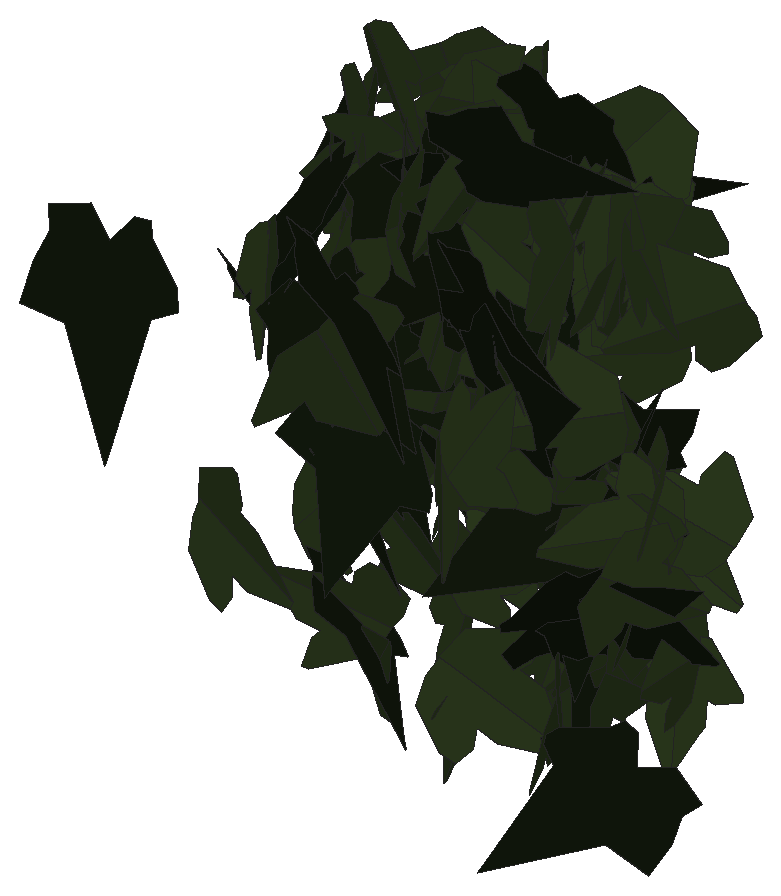
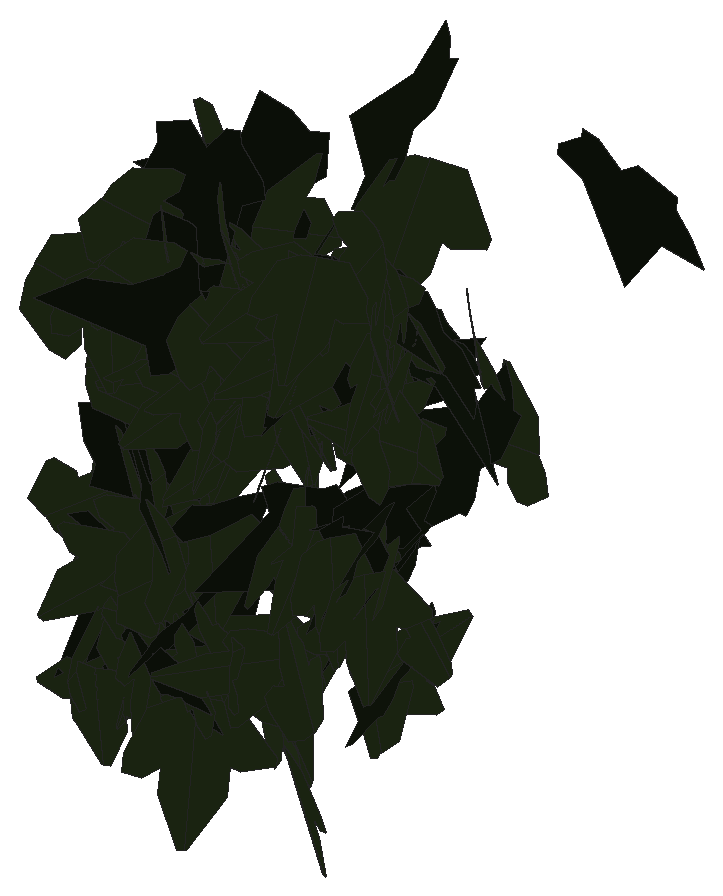
# SketchUp Ruby script. Lengths in inches.
U = 1.inch
M = Sketchup.active_model
def pt(a) = Geom::Point3d.new(a.map { |v| v * U })
def face(e, loops, mat)
  f = e.add_face(loops[0].map { |a| pt(a) })
  loops[1..].each { |l| e.add_face(l.map { |a| pt(a) }).erase! }
  f.material = f.back_material = mat if mat
  f
end
# faces: each face lists its corners as indices into pts; further lists are holes
def faces(e, pts, list, mat = nil) = list.each { |f| face(e, (f[0].is_a?(Array) ? f : [f]).map { |l| l.map { |i| pts[i] } }, mat) }
# xy, xz, yz: faces in a plane at the given z, y or x. An outline is a flat list of corners, or four numbers for a rectangle; further outlines are holes
def ring(l) = l.size == 4 ? [[l[0], l[1]], [l[2], l[1]], [l[2], l[3]], [l[0], l[3]]] : l.each_slice(2).to_a
def flat(e, list, mat, &to3) = list.each { |f| face(e, (f[0].is_a?(Array) ? f : [f]).map { |l| ring(l).map { |u, v| to3.(u, v) } }, mat) }
def xy(e, z, list, mat = nil) = flat(e, list, mat) { |x, y| [x, y, z] }
def xz(e, y, list, mat = nil) = flat(e, list, mat) { |x, z| [x, y, z] }
def yz(e, x, list, mat = nil) = flat(e, list, mat) { |y, z| [x, y, z] }
def lines(e, pts, list) = list.each { |a, b| e.add_line(pt(pts[a]), pt(pts[b])) }
# prism: a flat outline (further loops are holes) pulled along v
def prism(e, loops, v, mat = nil)
  f = face(e, loops, mat); d = Geom::Vector3d.new(v.map { |x| x * U })
  f.pushpull(f.normal.samedirection?(d) ? d.length : -d.length)
end
def box(e, o, s, mat = nil) = prism(e, [[o, [o[0] + s[0], o[1], o[2]], [o[0] + s[0], o[1] + s[1], o[2]], [o[0], o[1] + s[1], o[2]]]], [0, 0, s[2]], mat)
def at(x, y, z, deg = 0) = Geom::Transformation.translation(pt([x, y, z])) * Geom::Transformation.rotation(ORIGIN, Z_AXIS, deg.degrees)
def axes(o, x, y, z) = Geom::Transformation.new([*x, 0, *y, 0, *z, 0, *pt(o).to_a, 1])
def part(name) = M.definitions.add(name)
# library, detail: a bought-in or finely detailed component or shape, given as its bounding box
def library(name, o, s) = part(name).tap { |d| box(d.entities, o, s) }
def detail(e, o, s) = box(e.add_group.entities, o, s)
def put(e, d, t, mat = nil) = e.add_instance(d, t).tap { |i| i.material = mat if mat }
def group(e, t, mat = nil) = e.add_group.tap { |g| g.transformation = t; g.material = mat if mat }.entities
root = M.entities
M.materials.add("efeu1").color = [18, 25, 13]
M.materials.add("efeu2").color = [43, 57, 29]
c1 = part("ivyleaf_10")
p = [[0,0.5,-0.03],[-0.0625,2.02,-0.43],[-0.19,2.01,-0.46],[-0.54,1.05,-0.29],[-0.52,0.625,-0.18],[-0.83,0.76,-0.28],
  [-1.16,0.64,-0.33],[-1.15,0.33,-0.24],[-0.77,-0.39,0.02],[-0.3,-0.51,0.16],[0.04,-0.48,0.23],[-0.02,2.01,-0.4375],
  [-0.06,2.01,-0.43],[0.04,-0.49,0.23],[0.67,-0.49,0.14],[1.38,0.36,-0.2],[1.375,0.51,-0.24],[0.81,0.65,-0.19],
  [0.62,0.59,-0.15],[0.6,1.09,-0.28],[0.5,1.23,-0.31]]
faces(c1.entities,p,[[0,1,2,3,4,5,6,7,8,9,10],[11,12,0,13,14,15,16,17,18,19,20]],"efeu2")
c2 = part("ivyleaf_9")
p = [[1.54,2.16,1.25],[1.36,2.04,1.19],[-0.21,0.99,0.68],[-0.71,1.11,0.82],[-0.85,0.86,0.67],[-0.8,0.17,0.21],
  [-0.9,-0.01,0.1],[-0.67,-0.16,-0.02],[-0.08,-0.08,-0.05],[-0.03,-0.6,-0.4],[0.65,-0.88,-0.66],[0.83,-0.6,-0.49],
  [1.29,-0.42,-0.43],[1.8125,-0.07,-0.26],[1.21,0.44,0.15]]
faces(c2.entities,p,[[0,1,2,3,4,5,6,7,8,9,10,11,12,13,14]],"efeu1")
put(root,c1,axes([519.33,135.79,170.69],[-0.23266,0.62806,-0.07451],[0.02428,-0.07046,-0.66976],[-0.63199,-0.23391,0.0017]))
put(root,c1,axes([519.5,136.4375,167.12],[-0.25165,-0.66074,-0.04821],[0.01912,0.04431,-0.70703],[0.66222,-0.25237,0.00209]))
put(root,c1,axes([519.49,136.15,169.66],[-0.01709,-0.51856,0.5127],[0.02176,-0.51297,-0.51812],[0.7289,0.00315,0.02749]))
put(root,c1,axes([519.18,136.53,171.21],[0.40833,-0.42792,0.4417],[0.33385,-0.29103,-0.59058],[0.51648,0.52643,0.03254]))
put(root,c2,axes([519.73,134.51,170.41],[-0.53157,0.4474,-0.34863],[-0.26413,0.22758,0.69478],[0.50194,0.59357,-0.00361]))
put(root,c2,axes([518.93,134.71,168.71],[0.30061,-0.52854,0.55192],[0.33869,-0.43951,-0.60536],[0.68502,0.44924,0.05711]))
put(root,c2,axes([519.96,134.43,170.3],[-0.45095,0.63568,0.03637],[-0.02109,0.02963,-0.77938],[-0.63637,-0.45144,0.00006]))
put(root,c2,axes([519.4,130.97,171.44],[-0.62902,-0.2297,-0.64286],[0.60631,0.21376,-0.66963],[0.31374,-0.87364,0.00518]))
put(root,c1,axes([519.39,135.875,171.5],[-0.28758,0.30723,-0.51733],[0.2824,-0.43739,-0.41674],[-0.5313,-0.39878,0.05851]))
put(root,c1,axes([519.67,135.97,170.63],[-0.01143,-0.49947,-0.4386],[0.05584,0.4364,-0.49841],[0.66236,-0.04541,0.03445]))
put(root,c1,axes([519.42,134.04,170.125],[0.46577,-0.26689,0.42385],[0.35567,-0.2313,-0.53649],[0.35268,0.58574,-0.01872]))
put(root,c1,axes([519.34,135.15,165.76],[0.42672,-0.23414,-0.46095],[0.40158,-0.22632,0.48672],[-0.32562,-0.58596,-0.0038]))
put(root,c1,axes([519.28,136.04,169.49],[-0.02495,-0.08833,0.66389],[0.61696,0.25549,0.05717],[-0.26062,0.61327,0.0718]))
put(root,c1,axes([520.23,135.5,171.12],[0.3467,0.09818,-0.56949],[-0.57753,0.08246,-0.33738],[0.02053,0.66161,0.12656]))
put(root,c1,axes([519.9375,136.61,167.62],[-0.19817,-0.6743,-0.05006],[0.00873,0.04961,-0.70279],[0.6761,-0.19829,-0.0056]))
put(root,c1,axes([519.99,135.5625,169.02],[-0.38877,-0.52025,-0.20837],[-0.12833,-0.16422,0.64945],[-0.54554,0.40938,-0.00429]))
put(root,c1,axes([519.68,136,166.91],[-0.37064,0.21017,0.64179],[0.50889,-0.39435,0.42303],[0.44396,0.6275,0.05089]))
put(root,c1,axes([519.8125,136,172.27],[-0.4826,0.31295,-0.40914],[0.31544,-0.26367,-0.57377],[-0.40722,-0.57513,0.04042]))
put(root,c2,axes([519.75,135.83,166.98],[0.37466,-0.64244,-0.187],[-0.09447,0.16138,-0.7437],[0.6624,0.38638,-0.0003]))
put(root,c2,axes([520.1875,136.2,168.02],[-0.41218,-0.63662,0.24656],[-0.11009,-0.22226,-0.75792],[0.67377,-0.42577,0.02699]))
put(root,c1,axes([520.59,134.72,164.89],[-0.32035,-0.19606,-0.6035],[-0.51146,-0.32036,0.37557],[-0.37558,0.60349,0.0033]))
put(root,c2,axes([519.79,136.33,167.6],[0.42774,-0.61794,0.13653],[0.08201,-0.10927,-0.75153],[0.62751,0.4355,0.00516]))
put(root,c1,axes([520.25,136.72,171.97],[-0.43152,-0.5374,-0.18953],[0.13459,0.1349,-0.68893],[0.55373,-0.45159,0.01975]))
put(root,c1,axes([520.15,137,165.48],[0.19906,-0.67643,-0.07018],[0.03815,-0.0619,0.70486],[-0.67899,-0.20179,0.01903]))
put(root,c1,axes([519.83,136.18,166.74],[-0.24481,-0.21364,0.74665],[0.58059,0.4696,0.32472],[-0.51579,0.62999,0.01115]))
put(root,c1,axes([520.31,136.56,167.92],[-0.20784,-0.53843,-0.40911],[0.14041,0.38431,-0.57712],[0.66148,-0.25075,-0.00604]))
put(root,c1,axes([520.23,136.3,171.27],[-0.52379,-0.43811,-0.3686],[0.27047,0.25099,-0.68266],[0.50464,-0.58926,-0.01671]))
put(root,c1,axes([520.57,136.03,167.3],[-0.40169,-0.57434,0.1525],[-0.08114,-0.12933,-0.70083],[0.58868,-0.40973,0.00746]))
put(root,c1,axes([520.41,137.14,168.17],[-0.00629,0.59882,-0.47127],[-0.05118,-0.47056,-0.59723],[-0.76031,0.02672,0.0441]))
put(root,c2,axes([520.26,134.26,169.59],[0.17214,-0.5842,-0.53926],[-0.08366,0.53539,-0.60671],[0.79063,0.18384,0.05321]))
put(root,c2,axes([520.03,134.69,167.17],[0.42398,-0.59008,0.34279],[0.18551,-0.28871,-0.72643],[0.65673,0.46251,-0.01611]))
put(root,c1,axes([520.55,136.64,164.2],[0.5799,-0.53773,-0.01596],[-0.01344,0.00898,-0.79084],[0.5378,0.58005,-0.00255]))
put(root,c2,axes([520.14,136.29,167.96],[0.04751,-0.01877,-0.7655],[0.33342,0.69096,0.00375],[0.68933,-0.33292,0.05094]))
put(root,c2,axes([520.17,134.91,165.01],[0.34293,-0.66391,0.2397],[0.12675,-0.20423,-0.74702],[0.69438,0.36516,0.01799]))
put(root,c1,axes([520.53,134.8125,164.08],[-0.48234,0.13534,0.4645],[0.4358,-0.16334,0.50012],[0.21013,0.64941,0.02899]))
put(root,c1,axes([521.02,136.16,170],[0.58753,-0.19388,-0.2971],[-0.27123,0.125,-0.61795],[0.22867,0.6464,0.03039]))
put(root,c2,axes([520.65,135.58,171],[0.0571,-0.5406,-0.59781],[-0.08751,0.59161,-0.54334],[0.80123,0.10314,-0.01674]))
put(root,c1,axes([520.24,132.02,167.34],[0.15126,-0.04534,0.82537],[0.82533,-0.03832,-0.15336],[0.04591,0.83824,0.03764]))
put(root,c1,axes([520.62,136.52,171.72],[-0.52511,-0.03265,-0.43392],[0.43514,-0.04425,-0.52325],[-0.00311,-0.67976,0.0549]))
put(root,c1,axes([520.78,136.22,170.46],[0.00261,0.04743,0.71943],[0.04134,0.71825,-0.0475],[-0.71981,0.04142,-0.00012]))
put(root,c1,axes([520.72,135.35,171.3125],[-0.10421,0.29403,-0.60238],[0.20064,-0.56798,-0.31195],[-0.63957,-0.22609,0.00029]))
put(root,c1,axes([521.1,134.81,170.04],[-0.04828,-0.35832,0.57818],[-0.09626,-0.5702,-0.36142],[0.67336,-0.1072,-0.01021]))
put(root,c2,axes([520.83,134.53,167.74],[-0.18099,-0.75598,0.18495],[-0.02625,-0.18385,-0.77716],[0.77783,-0.18211,0.01681]))
put(root,c1,axes([521.15,134.71,170.73],[-0.08628,0.16478,0.66581],[-0.32591,0.58061,-0.18592],[-0.60352,-0.3371,0.00522]))
put(root,c1,axes([520.73,136.46,171.71],[-0.24232,-0.2459,-0.64819],[0.44152,0.47465,-0.34512],[0.53449,-0.50357,-0.00878]))
put(root,c2,axes([520.39,135.45,170.53],[0.26919,0.35615,-0.71425],[0.43465,0.56678,0.44643],[0.66939,-0.51125,-0.00265]))
put(root,c1,axes([521.29,135.26,169.54],[0.14655,-0.22206,-0.63963],[-0.29604,0.56755,-0.26487],[0.60892,0.32937,0.02517]))
put(root,c1,axes([521.49,134.66,166.05],[-0.40606,0.21039,-0.52397],[-0.49986,0.1662,0.45411],[0.26259,0.64173,0.05418]))
put(root,c2,axes([520.93,136.74,169.06],[-0.00659,-0.28089,0.71899],[-0.01168,-0.7189,-0.28096],[0.77182,-0.01327,0.00189]))
put(root,c1,axes([520.82,136.2,167.51],[0.02241,-0.05749,0.67477],[0.55204,-0.38952,-0.05152],[0.39227,0.55145,0.03395]))
put(root,c1,axes([521.31,136.14,167.93],[0.35311,-0.57726,-0.18258],[-0.09782,0.15419,-0.67669],[0.59749,0.3664,-0.00288]))
put(root,c2,axes([520.93,136.83,170.57],[0.14438,-0.73635,0.28054],[0.04963,-0.27615,-0.75037],[0.78642,0.15262,-0.00415]))
put(root,c1,axes([521.51,135.6,169.69],[-0.27167,-0.78398,0.10246],[-0.02615,-0.09937,-0.82968],[0.79021,-0.27282,0.00777]))
put(root,c1,axes([520.98,136.15,165.02],[-0.2513,-0.10464,0.59052],[0.5522,0.20942,0.2721],[-0.23397,0.60664,0.00793]))
put(root,c1,axes([521.88,136.28,168.89],[0.09787,0.35208,0.67435],[-0.27451,-0.61775,0.36237],[0.70947,-0.28759,0.04719]))
put(root,c1,axes([521.95,136.65,165.45],[0.41481,-0.11474,0.54991],[-0.5213,0.17609,0.42996],[-0.20932,-0.66593,0.01895]))
put(root,c1,axes([521.24,136.52,165.57],[0.16282,-0.1407,-0.73673],[0.58167,0.49964,0.03313],[0.47353,-0.56537,0.21262]))
put(root,c2,axes([521.48,135.14,169.55],[-0.17973,-0.10602,0.805],[0.68086,0.42953,0.20858],[-0.44238,0.70415,-0.00604]))
put(root,c1,axes([522.02,136.78,170.73],[-0.26971,-0.44167,0.43769],[-0.226,-0.37484,-0.5175],[0.57928,-0.35188,0.00189]))
put(root,c1,axes([521.62,136.79,172.21],[0.47707,-0.32733,0.41814],[0.33292,-0.25354,-0.57833],[0.4137,0.58151,-0.01678]))
put(root,c1,axes([521.74,134.85,167.43],[-0.1686,0.55926,-0.41859],[0.11803,-0.40161,-0.58412],[-0.68852,-0.2058,0.00237]))
put(root,c1,axes([521.92,135.29,164.2],[0.14994,-0.65208,0.19783],[0.04164,-0.19342,-0.66909],[0.68015,0.15559,-0.00265]))
put(root,c1,axes([521.83,135.52,171.71],[0.00181,-0.366,0.7582],[0.21242,-0.73347,-0.35457],[0.81468,0.19206,0.09077]))
put(root,c1,axes([522.16,135.9375,170.8125],[0.08029,0.14766,-0.67656],[-0.43865,-0.51618,-0.16471],[-0.53584,0.44468,0.03346]))
put(root,c1,axes([521.51,136.07,171.17],[-0.07759,-0.05338,-0.76196],[0.67215,-0.36856,-0.04262],[-0.36282,-0.67138,0.08398]))
put(root,c1,axes([522.23,135.92,169.26],[-0.15605,0.4272,0.60679],[-0.28096,0.53989,-0.45236],[-0.68685,-0.31791,0.04718]))
put(root,c2,axes([521.75,135.12,170.82],[0.45549,-0.63563,-0.11104],[-0.06315,0.09135,-0.78198],[0.64216,0.45984,0.00186]))
put(root,c1,axes([522.29,136.73,164.26],[-0.62581,-0.54341,-0.04469],[0.03437,0.02858,-0.82881],[0.54416,-0.62676,0.00095]))
put(root,c1,axes([522.17,131.91,170.6],[-0.3289,-0.76075,-0.42534],[0.20515,0.37428,-0.82805],[0.8471,-0.38601,0.03539]))
put(root,c1,axes([522.42,136.16,171.07],[0.75128,-0.00861,-0.03698],[-0.03689,0.00752,-0.75129],[0.00897,0.75215,0.00708]))
put(root,c1,axes([522.1875,134.67,164.59],[0.29857,0.42412,0.62452],[0.30949,0.54379,-0.51725],[-0.68856,0.42832,0.03831]))
put(root,c1,axes([522.69,135.91,166.86],[-0.54968,-0.45949,0.07673],[-0.06041,-0.04738,-0.71643],[0.46192,-0.55298,-0.00238]))
put(root,c1,axes([522.14,136.88,165.18],[0.3626,-0.17479,0.55642],[0.5525,-0.10693,-0.39363],[0.18682,0.65548,0.08416]))
put(root,c2,axes([522.89,136.05,166.71],[-0.47757,-0.42822,0.46382],[-0.35102,-0.30324,-0.6414],[0.52467,-0.59266,-0.00694]))
put(root,c1,axes([522.33,136.54,169.45],[-0.44851,-0.13524,-0.49031],[0.46838,0.14502,-0.46845],[0.19828,-0.64848,-0.00251]))
put(root,c1,axes([522.14,135.07,170.6875],[0.30306,0.07748,0.6264],[0.58938,0.21391,-0.31161],[-0.22585,0.66217,0.02737]))
put(root,c2,axes([522.84,135.77,172.67],[0.49521,0.23706,-0.52645],[-0.47962,-0.21721,-0.54897],[-0.32142,0.68935,0.00807]))
put(root,c2,axes([522.42,136.72,166.03],[0.0477,-0.81547,0.17255],[0.0191,-0.17172,-0.81681],[0.8333,0.05062,0.00884]))
put(root,c2,axes([522.71,135.41,170.07],[-0.67627,-0.11085,-0.41353],[0.40664,0.07549,-0.68525],[0.13391,-0.78908,-0.00747]))
put(root,c1,axes([522.25,136.54,169.72],[-0.18472,-0.05142,-0.72029],[0.70102,0.16566,-0.19161],[0.17331,-0.72491,0.0073]))
put(root,c2,axes([522.11,134.86,171.97],[0.44229,-0.04822,0.63431],[0.62875,-0.08427,-0.44482],[0.09668,0.76867,-0.00898]))
put(root,c1,axes([522.73,135.09,167.86],[0.03226,0.0851,0.77042],[-0.09607,0.76558,-0.08055],[-0.76913,-0.09206,0.04237]))
put(root,c1,axes([522.45,135.5,169.17],[-0.32877,-0.02586,-0.57333],[0.55372,-0.18805,-0.30904],[-0.15092,-0.63359,0.11512]))
put(root,c2,axes([522.83,136.86,165.24],[-0.63069,-0.076,-0.43592],[0.43041,0.07082,-0.63507],[0.10271,-0.7634,-0.01552]))
put(root,c2,axes([522.25,134.46,170.34],[0.28051,0.03211,-0.76052],[0.74445,0.15749,0.28123],[0.15877,-0.79516,0.02499]))
put(root,c1,axes([523.08,137.01,166.39],[-0.02062,-0.0121,-0.69439],[-0.31136,-0.62081,0.02006],[-0.62079,0.31177,0.013]))
put(root,c1,axes([523.21,134.14,169.72],[-0.47949,0.27866,0.43713],[-0.37524,0.22425,-0.55457],[-0.35767,-0.60885,-0.00419]))
put(root,c2,axes([522.42,136.48,170.83],[0.43552,0.06376,0.62922],[0.59113,0.23053,-0.43252],[-0.22481,0.72969,0.08166]))
put(root,c2,axes([522.37,131.89,171.55],[0.42721,-0.74552,0.44349],[0.2131,-0.38901,-0.85921],[0.84087,0.47735,-0.00757]))
put(root,c1,axes([523.11,135.16,169.8],[0.27733,-0.58945,-0.42413],[-0.11177,0.41395,-0.64839],[0.71753,0.29231,0.06293]))
put(root,c1,axes([523.28,137.04,171.2],[0.35853,0.26653,-0.51125],[-0.45856,-0.23309,-0.44311],[-0.34947,0.5793,0.05692]))
put(root,c1,axes([523.26,135.5,168.67],[-0.69559,-0.32197,0.17383],[-0.15751,-0.07355,-0.76649],[0.33026,-0.7132,0.00057]))
put(root,c1,axes([523.28,136.24,165.05],[-0.12375,-0.68789,-0.34855],[0.03114,0.34827,-0.69838],[0.77053,-0.12455,-0.02776]))
put(root,c1,axes([523.3,135.92,171.65],[0.22013,-0.63361,-0.1607],[-0.06452,0.14768,-0.67065],[0.65048,0.22906,-0.01214]))
put(root,c1,axes([523.5,136.8,172.09],[0.35545,0.30668,-0.53779],[-0.40065,-0.35881,-0.46942],[-0.47197,0.53555,-0.00654]))
put(root,c1,axes([523.59,136.35,165.32],[-0.20255,-0.43999,0.57486],[-0.25282,-0.51636,-0.48429],[0.67833,-0.32383,-0.00884]))
put(root,c1,axes([522.95,135.93,169.85],[0.50235,-0.11842,-0.47931],[0.47815,-0.05369,0.5144],[-0.12302,-0.69226,0.0421]))
put(root,c1,axes([523.03,136.73,166.92],[-0.44099,0.08158,-0.5989],[0.59048,-0.10023,-0.44844],[-0.12913,-0.73696,-0.00531]))
put(root,c2,axes([523.44,136.01,167.67],[0.59496,0.14798,0.48713],[-0.47334,-0.11512,0.61309],[0.18747,-0.76028,0.00198]))
put(root,c1,axes([523.63,136.95,170.72],[-0.58516,-0.33892,0.084],[-0.06804,-0.05012,-0.67616],[0.34248,-0.58903,0.00921]))
put(root,c2,axes([523.28,136.1,166.84],[-0.10287,0.57987,0.50112],[0.07788,-0.49509,0.58887],[0.76243,0.12881,0.00746]))
put(root,c1,axes([524.03,136.08,170.32],[-0.05063,0.0198,0.73075],[-0.69505,0.22566,-0.05427],[-0.2265,-0.69688,0.00319]))
put(root,c1,axes([523.89,136.46,169.22],[-0.03789,-0.00104,0.71493],[-0.36513,-0.61549,-0.02024],[0.61466,-0.36569,0.03204]))
put(root,c1,axes([523.69,134.55,164.76],[0.23288,-0.544,-0.47698],[-0.10198,0.4714,-0.58742],[0.71627,0.24398,0.07144]))
put(root,c2,axes([523.24,134.77,165.69],[0.10438,0.77359,-0.37329],[0.05044,0.36987,0.7806],[0.85747,-0.11592,-0.00047]))
put(root,c2,axes([523.14,134.22,169.1875],[0.08084,-0.10708,0.80382],[0.49618,-0.6324,-0.13415],[0.6414,0.50271,0.00246]))
put(root,c1,axes([523.83,135.66,170.67],[0.0673,-0.66352,-0.22259],[0.00471,0.22404,-0.66642],[0.69984,0.0623,0.02589]))
put(root,c1,axes([523.82,135.58,164.84],[0.09105,-0.46133,-0.60617],[0.03026,0.61219,-0.46137],[0.76115,0.03084,0.09085]))
put(root,c1,axes([523.87,135.89,165.0625],[0.21573,-0.34624,0.53241],[-0.23583,0.47841,0.40669],[-0.58968,-0.318,0.03214]))
put(root,c1,axes([523.5,136.21,167.5],[-0.46255,0.32518,-0.48346],[0.38598,-0.29139,-0.56528],[-0.43645,-0.60231,0.01246]))
put(root,c1,axes([523.64,135.67,171.5],[0.68684,-0.18781,0.22299],[0.21427,-0.06181,-0.71205],[0.1977,0.71948,-0.00296]))
put(root,c1,axes([523.54,132.98,169.01],[0.57186,-0.21838,-0.37785],[0.34957,-0.14367,0.61209],[-0.26128,-0.67019,-0.00809]))
put(root,c1,axes([524.1,136.05,167.71],[0.48192,-0.57651,-0.34397],[-0.22118,0.26343,-0.7514],[0.63384,0.53025,-0.00068]))
put(root,c1,axes([524.39,134.5,169.26],[-0.12783,-0.02624,0.7514],[-0.49612,-0.56976,-0.10429],[0.56494,-0.50628,0.07843]))
put(root,c1,axes([523.86,135.5,167.09],[-0.62066,-0.27224,-0.27051],[0.25435,0.09338,-0.67757],[0.2874,-0.67058,0.01547]))
put(root,c1,axes([523.54,136.68,166.34],[0.33873,0.28691,0.5898],[0.4568,0.37315,-0.44386],[-0.47065,0.56865,-0.00632]))
put(root,c1,axes([523.85,136.84,164.48],[0.68546,0.17596,0.05789],[0.05624,0.01372,-0.70768],[-0.17649,0.68776,-0.00069]))
put(root,c2,axes([523.83,135.18,165.82],[0.58644,0.51336,0.23414],[0.1736,0.15716,-0.77938],[-0.53687,0.61158,0.00374]))
put(root,c1,axes([524.27,133.93,171.73],[0.53524,-0.52888,-0.44565],[-0.27859,0.3509,-0.75103],[0.63301,0.60162,0.04628]))
put(root,c1,axes([524.3,135.8,166.98],[-0.0375,0.11701,0.77345],[-0.16456,-0.75819,0.10673],[0.76475,-0.15741,0.06089]))
put(root,c1,axes([524.11,136.82,164.65],[-0.10806,0.12708,0.71764],[0.32239,-0.64231,0.16228],[0.65362,0.33782,0.0386]))
put(root,c1,axes([524.65,136.5,166.78],[0.23205,0.33033,0.58383],[-0.42147,-0.40881,0.39882],[0.52186,-0.47705,0.0625]))
put(root,c1,axes([524.35,135.51,171.27],[-0.24087,0.69085,0.26597],[-0.09098,0.24995,-0.73163],[-0.73467,-0.25746,0.0034]))
put(root,c2,axes([524.74,134.82,164.08],[0.01522,0.0354,-0.79946],[-0.19367,-0.77567,-0.03804],[-0.77645,0.19417,-0.00619]))
put(root,c1,axes([524.94,136.32,170.19],[-0.25578,-0.2451,0.72492],[-0.54577,-0.47734,-0.35396],[0.53639,-0.60256,-0.01446]))
put(root,c1,axes([524.29,135.16,166.55],[-0.18866,-0.40508,-0.63403],[0.3428,0.5356,-0.44419],[0.66976,-0.38824,0.04875]))
